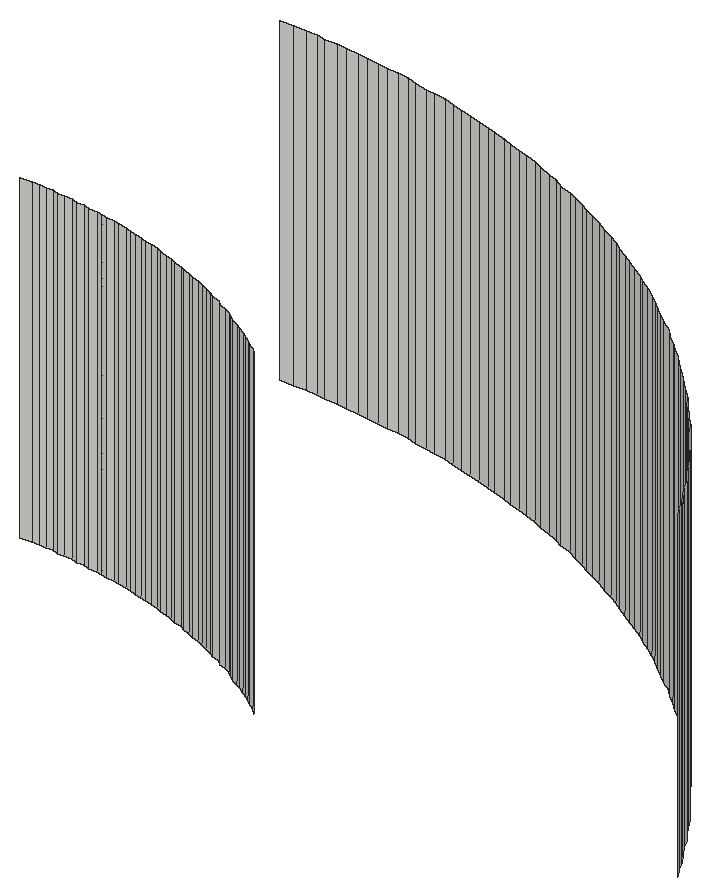
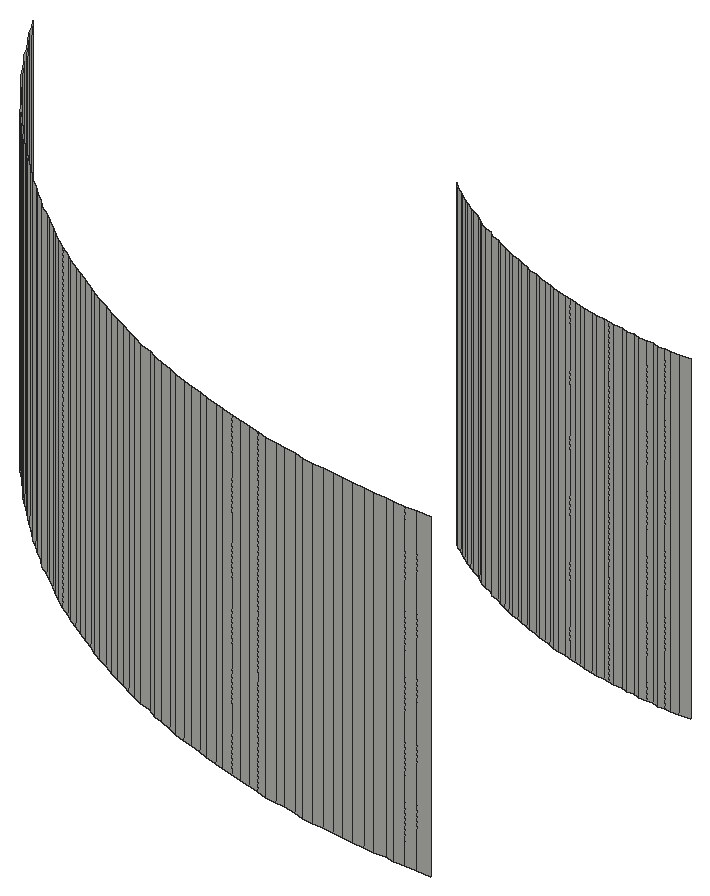
# SketchUp Ruby script. Lengths in inches.
U = 1.inch
M = Sketchup.active_model
def pt(a) = Geom::Point3d.new(a.map { |v| v * U })
def face(e, loops, mat)
  f = e.add_face(loops[0].map { |a| pt(a) })
  loops[1..].each { |l| e.add_face(l.map { |a| pt(a) }).erase! }
  f.material = f.back_material = mat if mat
  f
end
# faces: each face lists its corners as indices into pts; further lists are holes
def faces(e, pts, list, mat = nil) = list.each { |f| face(e, (f[0].is_a?(Array) ? f : [f]).map { |l| l.map { |i| pts[i] } }, mat) }
# xy, xz, yz: faces in a plane at the given z, y or x. An outline is a flat list of corners, or four numbers for a rectangle; further outlines are holes
def ring(l) = l.size == 4 ? [[l[0], l[1]], [l[2], l[1]], [l[2], l[3]], [l[0], l[3]]] : l.each_slice(2).to_a
def flat(e, list, mat, &to3) = list.each { |f| face(e, (f[0].is_a?(Array) ? f : [f]).map { |l| ring(l).map { |u, v| to3.(u, v) } }, mat) }
def xy(e, z, list, mat = nil) = flat(e, list, mat) { |x, y| [x, y, z] }
def xz(e, y, list, mat = nil) = flat(e, list, mat) { |x, z| [x, y, z] }
def yz(e, x, list, mat = nil) = flat(e, list, mat) { |y, z| [x, y, z] }
def lines(e, pts, list) = list.each { |a, b| e.add_line(pt(pts[a]), pt(pts[b])) }
# prism: a flat outline (further loops are holes) pulled along v
def prism(e, loops, v, mat = nil)
  f = face(e, loops, mat); d = Geom::Vector3d.new(v.map { |x| x * U })
  f.pushpull(f.normal.samedirection?(d) ? d.length : -d.length)
end
def box(e, o, s, mat = nil) = prism(e, [[o, [o[0] + s[0], o[1], o[2]], [o[0] + s[0], o[1] + s[1], o[2]], [o[0], o[1] + s[1], o[2]]]], [0, 0, s[2]], mat)
def at(x, y, z, deg = 0) = Geom::Transformation.translation(pt([x, y, z])) * Geom::Transformation.rotation(ORIGIN, Z_AXIS, deg.degrees)
def axes(o, x, y, z) = Geom::Transformation.new([*x, 0, *y, 0, *z, 0, *pt(o).to_a, 1])
def part(name) = M.definitions.add(name)
# library, detail: a bought-in or finely detailed component or shape, given as its bounding box
def library(name, o, s) = part(name).tap { |d| box(d.entities, o, s) }
def detail(e, o, s) = box(e.add_group.entities, o, s)
def put(e, d, t, mat = nil) = e.add_instance(d, t).tap { |i| i.material = mat if mat }
def group(e, t, mat = nil) = e.add_group.tap { |g| g.transformation = t; g.material = mat if mat }.entities
root = M.entities
xz(root,174.2,[[144.55,121,144.59,123]])
xz(root,174.22,[[144.42,121,144.47,123]])
xz(root,174.23,[[144.34,121,144.38,123]])
xz(root,174.24,[[144.21,121,144.25,123],[144.25,121,144.3,123]])
xz(root,174.25,[[143.97,121,144.04,123],[144.04,121,144.09,123],[144.09,121,144.13,123],[144.13,121,144.17,123]])
xz(root,176.2,[[144.69,121,144.75,123]])
xz(root,176.23,[[144.41,121,144.48,123]])
xz(root,176.24,[[144.27,121,144.34,123]])
xz(root,176.25,[[143.98,121,144.07,123],[144.07,121,144.14,123],[144.14,121,144.21,123]])
p = [[145.91,173.63,121],[145.94,173.6,121],[145.94,173.6,123],[145.91,173.63,123],[145.875,173.65,121],[145.875,173.65,123],
  [148.55,173.625,121],[148.51,173.68,121],[148.51,173.68,123],[148.55,173.625,123],[145.73,173.75,121],[145.77,173.73,121],
  [145.77,173.73,123],[145.73,173.75,123],[145.7,173.77,121],[145.7,173.77,123],[145.84,173.68,121],[145.84,173.68,123],
  [145.81,173.7,121],[145.81,173.7,123],[148.48,173.74,121],[148.44,173.8,121],[148.44,173.8,123],[148.48,173.74,123],
  [145.625,173.8125,121],[145.66,173.79,121],[145.66,173.79,123],[145.625,173.8125,123],[145.59,173.84,121],[145.59,173.84,123],
  [145.55,173.86,121],[145.55,173.86,123],[148.4,173.86,121],[148.4,173.86,123],[145.4375,173.91,121],[145.48,173.9,121],
  [145.48,173.9,123],[145.4375,173.91,123],[145.4,173.93,121],[145.4,173.93,123],[145.36,173.95,121],[145.36,173.95,123],
  [145.51,173.875,121],[145.51,173.875,123],[148.37,173.92,121],[148.33,173.97,121],[148.33,173.97,123],[148.37,173.92,123],
  [145.125,174.05,121],[145.16,174.03,121],[145.16,174.03,123],[145.125,174.05,123],[145.08,174.0625,121],[145.08,174.0625,123],
  [145.24,174,121],[145.28,173.99,121],[145.28,173.99,123],[145.24,174,123],[145.2,174.02,121],[145.2,174.02,123],
  [145.32,173.97,121],[145.32,173.97,123],[148.29,174.03,121],[148.25,174.09,121],[148.25,174.09,123],[148.29,174.03,123],
  [144.84,174.14,121],[144.88,174.13,121],[144.88,174.13,123],[144.84,174.14,123],[144.8,174.15,121],[144.8,174.15,123],
  [144.76,174.16,121],[144.76,174.16,123],[144.92,174.12,121],[144.96,174.1,121],[144.96,174.1,123],[144.92,174.12,123],
  [145.04,174.08,121],[145.04,174.08,123],[145,174.09,121],[145,174.09,123],[148.21,174.14,121],[148.21,174.14,123],
  [148.16,174.2,121],[148.16,174.2,123],[144.17,174.25,121],[144.21,174.24,121],[144.21,174.24,123],[144.17,174.25,123],
  [144.3,174.24,121],[144.34,174.23,121],[144.34,174.23,123],[144.3,174.24,123],[144.38,174.23,121],[144.42,174.22,121],
  [144.42,174.22,123],[144.38,174.23,123],[144.51,174.21,121],[144.55,174.2,121],[144.55,174.2,123],[144.51,174.21,123],
  [144.47,174.22,121],[144.47,174.22,123],[144.63,174.1875,121],[144.68,174.18,121],[144.68,174.18,123],[144.63,174.1875,123],
  [144.59,174.2,121],[144.59,174.2,123],[144.72,174.17,121],[144.72,174.17,123],[148.12,174.25,121],[148.12,174.25,123],
  [148.08,174.3,121],[148.04,174.36,121],[148.04,174.36,123],[148.08,174.3,123],[147.99,174.41,121],[147.95,174.46,121],
  [147.95,174.46,123],[147.99,174.41,123],[147.9,174.51,121],[147.9,174.51,123],[147.86,174.5625,121],[147.86,174.5625,123],
  [147.81,174.61,121],[147.81,174.61,123],[147.76,174.66,121],[147.76,174.66,123],[147.71,174.71,121],[147.71,174.71,123],
  [147.66,174.76,121],[147.66,174.76,123],[147.61,174.81,121],[147.61,174.81,123],[147.5625,174.86,121],[147.5625,174.86,123],
  [147.46,174.95,121],[147.41,174.99,121],[147.41,174.99,123],[147.46,174.95,123],[147.51,174.9,121],[147.51,174.9,123],
  [147.36,175.04,121],[147.3,175.08,121],[147.3,175.08,123],[147.36,175.04,123],[147.25,175.12,121],[147.2,175.16,121],
  [147.2,175.16,123],[147.25,175.12,123],[147.09,175.25,121],[147.03,175.29,121],[147.03,175.29,123],[147.09,175.25,123],
  [147.14,175.21,121],[147.14,175.21,123],[146.97,175.33,121],[146.92,175.37,121],[146.92,175.37,123],[146.97,175.33,123],
  [146.8,175.44,121],[146.74,175.48,121],[146.74,175.48,123],[146.8,175.44,123],[146.86,175.4,121],[146.86,175.4,123],
  [146.68,175.51,121],[146.625,175.55,121],[146.625,175.55,123],[146.68,175.51,123],[146.57,175.58,121],[146.57,175.58,123],
  [146.51,175.61,121],[146.44,175.65,121],[146.44,175.65,123],[146.51,175.61,123],[146.38,175.68,121],[146.38,175.68,123],
  [146.26,175.74,121],[146.2,175.77,121],[146.2,175.77,123],[146.26,175.74,123],[146.32,175.71,121],[146.32,175.71,123],
  [146.07,175.82,121],[146.01,175.85,121],[146.01,175.85,123],[146.07,175.82,123],[146.14,175.8,121],[146.14,175.8,123],
  [145.75,175.95,121],[145.6875,175.97,121],[145.6875,175.97,123],[145.75,175.95,123],[145.88,175.9,121],[145.82,175.93,121],
  [145.82,175.93,123],[145.88,175.9,123],[145.95,175.875,121],[145.95,175.875,123],[145.49,176.03,121],[145.43,176.05,121],
  [145.43,176.05,123],[145.49,176.03,123],[145.56,176.01,121],[145.56,176.01,123],[145.62,175.99,121],[145.62,175.99,123],
  [145.09,176.14,121],[145.02,176.15,121],[145.02,176.15,123],[145.09,176.14,123],[144.96,176.16,121],[144.96,176.16,123],
  [145.16,176.12,121],[145.16,176.12,123],[145.29,176.09,121],[145.23,176.1,121],[145.23,176.1,123],[145.29,176.09,123],
  [145.36,176.07,121],[145.36,176.07,123],[144.27,176.24,121],[144.21,176.25,121],[144.21,176.25,123],[144.27,176.24,123],
  [144.41,176.23,121],[144.34,176.24,121],[144.34,176.24,123],[144.41,176.23,123],[144.62,176.21,121],[144.55,176.22,121],
  [144.55,176.22,123],[144.62,176.21,123],[144.48,176.23,121],[144.48,176.23,123],[144.69,176.2,121],[144.69,176.2,123],
  [144.89,176.17,121],[144.82,176.19,121],[144.82,176.19,123],[144.89,176.17,123],[144.75,176.2,121],[144.75,176.2,123]]
faces(root,p,[[0,1,2,3],[4,0,3,5],[6,7,8,9],[10,11,12,13],[14,10,13,15],[16,4,5,17],[18,16,17,19],[11,18,19,12],
  [20,21,22,23],[7,20,23,8],[24,25,26,27],[28,24,27,29],[30,28,29,31],[25,14,15,26],[21,32,33,22],[34,35,36,37],
  [38,34,37,39],[40,38,39,41],[42,30,31,43],[35,42,43,36],[44,45,46,47],[32,44,47,33],[48,49,50,51],[52,48,51,53],
  [54,55,56,57],[58,54,57,59],[49,58,59,50],[60,40,41,61],[55,60,61,56],[62,63,64,65],[45,62,65,46],[66,67,68,69],
  [70,66,69,71],[72,70,71,73],[74,75,76,77],[67,74,77,68],[78,52,53,79],[80,78,79,81],[75,80,81,76],[63,82,83,64],
  [82,84,85,83],[86,87,88,89],[90,91,92,93],[94,95,96,97],[98,99,100,101],[102,98,101,103],[104,105,106,107],[108,104,107,109],
  [110,72,73,111],[105,110,111,106],[84,112,113,85],[114,115,116,117],[112,114,117,113],[118,119,120,121],[115,118,121,116],[119,122,123,120],
  [122,124,125,123],[124,126,127,125],[126,128,129,127],[128,130,131,129],[130,132,133,131],[132,134,135,133],[134,136,137,135],[138,139,140,141],
  [136,142,143,137],[142,138,141,143],[144,145,146,147],[139,144,147,140],[148,149,150,151],[145,148,151,146],[152,153,154,155],[149,156,157,150],
  [156,152,155,157],[158,159,160,161],[153,158,161,154],[162,163,164,165],[166,162,165,167],[159,166,167,160],[168,169,170,171],[169,172,173,170],
  [163,168,171,164],[174,175,176,177],[175,178,179,176],[172,174,177,173],[180,181,182,183],[178,184,185,179],[184,180,183,185],[186,187,188,189],
  [181,190,191,182],[190,186,189,191],[192,193,194,195],[196,197,198,199],[197,192,195,198],[187,200,201,188],[200,196,199,201],[202,203,204,205],
  [206,202,205,207],[193,208,209,194],[208,206,207,209],[210,211,212,213],[211,214,215,212],[216,210,213,217],[218,219,220,221],[219,216,217,220],
  [222,218,221,223],[203,222,223,204],[224,225,226,227],[228,229,230,231],[232,233,234,235],[233,236,237,234],[238,232,235,239],[240,241,242,243],
  [241,244,245,242],[214,240,243,215]])
